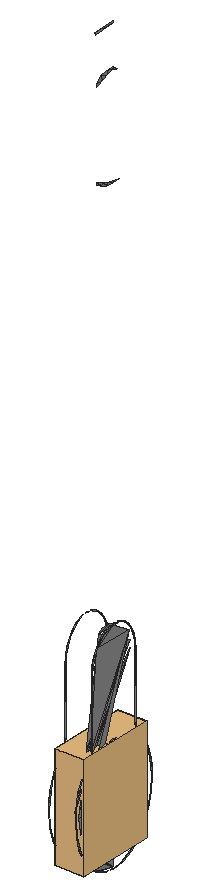
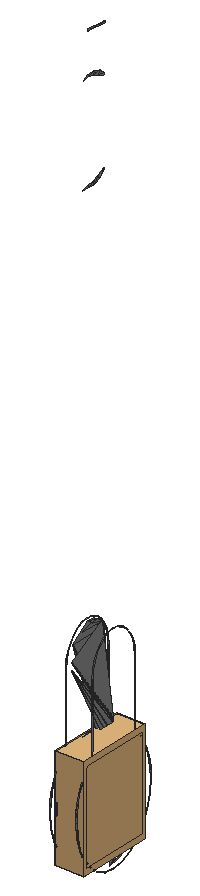
# SketchUp Ruby script. Lengths in inches.
U = 1.inch
M = Sketchup.active_model
def pt(a) = Geom::Point3d.new(a.map { |v| v * U })
def face(e, loops, mat)
  f = e.add_face(loops[0].map { |a| pt(a) })
  loops[1..].each { |l| e.add_face(l.map { |a| pt(a) }).erase! }
  f.material = f.back_material = mat if mat
  f
end
# faces: each face lists its corners as indices into pts; further lists are holes
def faces(e, pts, list, mat = nil) = list.each { |f| face(e, (f[0].is_a?(Array) ? f : [f]).map { |l| l.map { |i| pts[i] } }, mat) }
# xy, xz, yz: faces in a plane at the given z, y or x. An outline is a flat list of corners, or four numbers for a rectangle; further outlines are holes
def ring(l) = l.size == 4 ? [[l[0], l[1]], [l[2], l[1]], [l[2], l[3]], [l[0], l[3]]] : l.each_slice(2).to_a
def flat(e, list, mat, &to3) = list.each { |f| face(e, (f[0].is_a?(Array) ? f : [f]).map { |l| ring(l).map { |u, v| to3.(u, v) } }, mat) }
def xy(e, z, list, mat = nil) = flat(e, list, mat) { |x, y| [x, y, z] }
def xz(e, y, list, mat = nil) = flat(e, list, mat) { |x, z| [x, y, z] }
def yz(e, x, list, mat = nil) = flat(e, list, mat) { |y, z| [x, y, z] }
def lines(e, pts, list) = list.each { |a, b| e.add_line(pt(pts[a]), pt(pts[b])) }
# prism: a flat outline (further loops are holes) pulled along v
def prism(e, loops, v, mat = nil)
  f = face(e, loops, mat); d = Geom::Vector3d.new(v.map { |x| x * U })
  f.pushpull(f.normal.samedirection?(d) ? d.length : -d.length)
end
def box(e, o, s, mat = nil) = prism(e, [[o, [o[0] + s[0], o[1], o[2]], [o[0] + s[0], o[1] + s[1], o[2]], [o[0], o[1] + s[1], o[2]]]], [0, 0, s[2]], mat)
def at(x, y, z, deg = 0) = Geom::Transformation.translation(pt([x, y, z])) * Geom::Transformation.rotation(ORIGIN, Z_AXIS, deg.degrees)
def axes(o, x, y, z) = Geom::Transformation.new([*x, 0, *y, 0, *z, 0, *pt(o).to_a, 1])
def part(name) = M.definitions.add(name)
# library, detail: a bought-in or finely detailed component or shape, given as its bounding box
def library(name, o, s) = part(name).tap { |d| box(d.entities, o, s) }
def detail(e, o, s) = box(e.add_group.entities, o, s)
def put(e, d, t, mat = nil) = e.add_instance(d, t).tap { |i| i.material = mat if mat }
def group(e, t, mat = nil) = e.add_group.tap { |g| g.transformation = t; g.material = mat if mat }.entities
root = M.entities
M.materials.add("Material \#1").color = [140, 140, 140]
c1 = library("3DGeom~13_Defintion",[-84.91,-744.98,-830.03],[169.82,169.83,1000])
c2 = library("3DGeom~12_Defintion",[-95.68,-755.75,-830.03],[191.36,191.37,1000])
c3 = part("3DGeom~10_Defintion")
yz(c3.entities,-68.96,[[-797.08,-844.83,-797.08,-827.59,-922.41,-827.59],[-922.41,-844.83,-797.08,-844.83,-922.41,-827.59]],"Material \#1")
yz(c3.entities,68.97,[[-922.41,-844.83,-797.08,-827.59,-797.08,-844.83],[-922.41,-844.83,-922.41,-827.59,-797.08,-827.59],[-797.08,137.93,-922.41,155.17,-797.08,155.17],[-922.41,137.93,-922.41,155.17,-797.08,137.93]],"Material \#1")
p = [[-15.8,-989.55,-844.83],[-15.8,-989.55,-827.59],[0,-991.38,-827.59],[0,-991.38,-844.83],[15.8,-989.55,-827.59],[15.8,-989.55,-844.83],
  [-30.32,-984.36,-844.83],[-30.32,-984.36,-827.59],[30.31,-984.36,-827.59],[30.31,-984.36,-844.83],[-43.12,-976.21,-844.83],[-43.12,-976.21,-827.59],
  [43.12,-976.21,-827.59],[43.12,-976.21,-844.83],[-53.81,-965.53,-844.83],[-53.81,-965.53,-827.59],[53.8,-965.53,-827.59],[53.8,-965.53,-844.83],
  [-61.95,-952.73,-844.83],[-61.95,-952.73,-827.59],[53.8,-965.53,-827.59],[61.95,-952.73,-827.59],[61.95,-952.73,-844.83],[-67.15,-938.21,-844.83],
  [-67.15,-938.21,-827.59],[67.14,-938.21,-827.59],[67.14,-938.21,-844.83],[-68.96,-922.41,-844.83],[-68.96,-922.41,-827.59],[67.14,-938.21,-827.59],
  [68.97,-922.41,-827.59],[68.97,-922.41,-844.83],[-69.1,-794.86,-844.83],[-69.1,-794.86,-827.59],[-68.96,-797.08,-827.59],[-68.96,-797.08,-844.83],
  [68.97,-797.08,-844.83],[68.97,-797.08,-827.59],[69.11,-794.71,-827.59],[69.11,-794.71,-844.83],[-69.48,-792.73,-844.83],[-69.48,-792.73,-827.59],
  [69.53,-792.51,-827.59],[69.53,-792.51,-844.83],[-70.14,-790.6875,-844.83],[-70.14,-790.6875,-827.59],[70.24,-790.48,-827.59],[70.24,-790.48,-844.83],
  [-71.08,-788.73,-844.83],[-71.08,-788.73,-827.59],[71.22,-788.57,-827.59],[71.22,-788.57,-844.83],[-72.32,-786.86,-844.83],[-72.32,-786.86,-827.59],
  [72.47,-786.78,-827.59],[72.47,-786.78,-844.83],[-73.8,-785.17,-844.83],[-73.8,-785.17,-827.59],[74,-785.04,-827.59],[74,-785.04,-844.83],
  [-75.96,-783.21,-844.83],[-75.96,-783.21,-827.59],[74,-785.04,-827.59],[75.76,-783.39,-827.59],[75.76,-783.39,-844.83],[86.625,-772.95,-827.59],
  [86.61,-772.96,-844.83],[-86.89,-773.25,-844.83],[-86.89,-773.25,-827.59],[-75.96,-783.21,-844.83],[-96.66,-761.8,-844.83],[-96.66,-761.8,-827.59],
  [86.625,-772.95,-827.59],[86.63,-772.94,-844.83],[86.61,-772.96,-844.83],[86.625,-772.95,-827.59],[86.62,-772.95,-827.59],[86.62,-772.95,-827.59],
  [96.31,-761.375,-827.59],[96.31,-761.375,-844.83],[86.63,-772.94,-844.83],[86.625,-772.95,-827.59],[86.62,-772.95,-827.59],[-104.96,-749.18,-844.83],
  [-104.96,-749.18,-827.59],[-96.66,-761.8,-827.59],[-96.66,-761.8,-844.83],[96.31,-761.375,-827.59],[104.62,-748.77,-827.59],[104.62,-748.77,-844.83],
  [-111.64,-735.52,-844.83],[-111.64,-735.52,-827.59],[111.39,-735.21,-827.59],[111.39,-735.21,-844.83],[-116.49,-721.23,-844.83],[-116.49,-721.23,-827.59],
  [116.4375,-720.78,-827.59],[116.4375,-720.78,-844.83],[-119.64,-705.62,-844.83],[-119.64,-705.62,-827.59],[119.6,-705.57,-827.59],[119.6,-705.57,-844.83],
  [-120.6875,-689.65,-844.83],[-120.6875,-689.65,-827.59],[120.69,-689.65,-827.59],[120.69,-689.65,-844.83],[-117.5,-662,-844.83],[-117.5,-662,-827.59],
  [117.5,-662,-827.59],[117.5,-662,-844.83],[-108.41,-636.61,-844.83],[-108.41,-636.61,-827.59],[117.5,-662,-844.83],[108.41,-636.61,-827.59],
  [108.41,-636.61,-844.83],[-93.91,-613.95,-844.83],[-93.91,-613.95,-827.59],[-108.41,-636.61,-827.59],[108.41,-636.61,-844.83],[94.16,-614.19,-827.59],
  [94.16,-614.19,-844.83],[94.16,-614.19,-827.59],[75.46,-595.5,-827.59],[75.46,-595.5,-844.83],[-75.46,-595.5,-844.83],[-75.46,-595.5,-827.59],
  [-93.91,-613.95,-827.59],[-93.91,-613.95,-827.59],[-93.91,-613.95,-844.83],[-53.05,-581.24,-844.83],[-53.05,-581.24,-827.59],[-75.46,-595.5,-827.59],
  [-75.46,-595.5,-844.83],[53.05,-581.24,-827.59],[53.05,-581.24,-844.83],[-27.65,-572.16,-844.83],[-27.65,-572.16,-827.59],[-53.05,-581.24,-827.59],
  [-53.05,-581.24,-844.83],[27.66,-572.16,-827.59],[27.66,-572.16,-844.83],[0,-568.97,-844.83],[0,-568.97,-827.59],[-27.65,-572.16,-827.59],
  [-27.65,-572.16,-844.83],[0,-568.97,-844.83],[-15.8,-989.55,155.17],[0,-991.38,155.17],[0,-991.38,137.93],[-15.8,-989.55,137.93],
  [15.8,-989.55,155.17],[15.8,-989.55,137.93],[-30.32,-984.36,155.17],[-30.32,-984.36,137.93],[30.31,-984.36,155.17],[30.31,-984.36,137.93],
  [-43.125,-976.22,155.17],[-43.125,-976.22,137.93],[43.12,-976.22,155.17],[43.12,-976.22,137.93],[-53.81,-965.53,155.17],[-53.81,-965.53,137.93],
  [53.8,-965.53,155.17],[53.8,-965.53,137.93],[-61.96,-952.73,155.17],[-61.95,-952.73,137.93],[61.95,-952.73,155.17],[61.95,-952.73,137.93],
  [53.8,-965.53,137.93],[-67.15,-938.21,155.17],[-67.15,-938.21,137.93],[67.14,-938.21,155.17],[67.14,-938.21,137.93],[-68.96,-922.41,155.17],
  [-68.96,-922.41,137.93],[68.97,-922.41,155.17],[68.97,-922.41,137.93],[67.14,-938.21,137.93],[-68.97,-797.08,155.17],[-68.97,-797.08,137.93],
  [-69.1,-794.86,155.17],[-69.1,-794.86,137.93],[68.97,-797.08,155.17],[69.11,-794.71,155.17],[69.11,-794.71,137.93],[68.97,-797.08,137.93],
  [-69.48,-792.73,155.17],[-69.48,-792.73,137.93],[69.53,-792.51,155.17],[69.53,-792.51,137.93],[-70.14,-790.6875,155.17],[-70.14,-790.6875,137.93],
  [70.24,-790.48,155.17],[70.24,-790.48,137.93],[-71.08,-788.73,155.17],[-71.08,-788.73,137.93],[71.22,-788.57,155.17],[71.22,-788.57,137.93],
  [-72.32,-786.86,155.17],[-72.32,-786.86,137.93],[72.47,-786.78,155.17],[72.47,-786.78,137.93],[-73.8,-785.17,155.17],[-73.8,-785.17,137.93],
  [74,-785.04,155.17],[74,-785.04,137.93],[-75.96,-783.21,155.17],[-75.96,-783.21,137.93],[75.76,-783.39,155.17],[75.76,-783.39,137.93],
  [74,-785.04,137.93],[86.61,-772.96,155.17],[86.625,-772.95,137.93],[-86.88,-773.25,155.17],[-75.96,-783.21,155.17],[-86.88,-773.25,137.93],
  [-96.66,-761.8,155.17],[-96.66,-761.8,137.93],[86.63,-772.94,155.17],[86.625,-772.95,137.93],[86.61,-772.96,155.17],[86.62,-772.95,137.93],
  [86.625,-772.95,137.93],[96.31,-761.375,155.17],[96.31,-761.375,137.93],[86.62,-772.95,137.93],[86.63,-772.94,155.17],[86.62,-772.95,137.93],
  [86.625,-772.95,137.93],[-104.96,-749.18,155.17],[-96.66,-761.8,155.17],[-96.66,-761.8,137.93],[-104.96,-749.18,137.93],[104.62,-748.77,155.17],
  [104.62,-748.77,137.93],[96.31,-761.375,137.93],[-111.64,-735.52,155.17],[-111.64,-735.52,137.93],[111.39,-735.21,155.17],[111.39,-735.21,137.93],
  [-116.49,-721.23,155.17],[-116.49,-721.23,137.93],[116.4375,-720.78,155.17],[116.4375,-720.78,137.93],[-119.64,-705.62,155.17],[-119.64,-705.62,137.93],
  [119.6,-705.57,155.17],[119.6,-705.57,137.93],[-120.6875,-689.65,155.17],[-120.6875,-689.65,137.93],[120.69,-689.65,155.17],[120.69,-689.65,137.93],
  [-117.5,-662,155.17],[-117.5,-662,137.93],[117.5,-662,155.17],[117.5,-662,137.93],[-108.41,-636.61,155.17],[-108.41,-636.61,137.93],
  [117.5,-662,155.17],[108.41,-636.61,155.17],[108.41,-636.61,137.93],[-93.91,-613.95,155.17],[-108.41,-636.61,137.93],[-93.91,-613.95,137.93],
  [108.41,-636.61,155.17],[94.16,-614.19,155.17],[94.16,-614.19,137.93],[75.46,-595.5,155.17],[75.46,-595.5,137.93],[94.16,-614.19,137.93],
  [-75.46,-595.5,155.17],[-93.91,-613.95,155.17],[-93.91,-613.95,137.93],[-75.46,-595.5,137.93],[-53.05,-581.24,155.17],[-75.46,-595.5,155.17],
  [-75.46,-595.5,137.93],[-53.05,-581.24,137.93],[53.05,-581.24,155.17],[53.05,-581.24,137.93],[-27.65,-572.16,155.17],[-53.05,-581.24,155.17],
  [-53.05,-581.24,137.93],[-27.65,-572.16,137.93],[27.65,-572.16,155.17],[27.65,-572.16,137.93],[0,-568.97,155.17],[-27.65,-572.16,155.17],
  [-27.65,-572.16,137.93],[0,-568.97,137.93],[0,-568.97,155.17]]
faces(c3.entities,p,[[0,1,2],[2,3,0],[3,2,4],[4,5,3],[6,7,1],[1,0,6],[5,4,8],[8,9,5],
  [10,11,7],[7,6,10],[9,8,12],[12,13,9],[14,15,11],[11,10,14],[13,12,16],[16,17,13],
  [18,19,15],[15,14,18],[17,20,21],[21,22,17],[23,24,19],[19,18,23],[22,21,25],[25,26,22],
  [27,28,24],[24,23,27],[26,29,30],[30,31,26],[32,33,34],[34,35,32],[36,37,38],[38,39,36],
  [40,41,33],[33,32,40],[39,38,42],[42,43,39],[44,45,41],[41,40,44],[43,42,46],[46,47,43],
  [48,49,45],[45,44,48],[47,46,50],[50,51,47],[52,53,49],[49,48,52],[51,50,54],[54,55,51],
  [56,57,53],[53,52,56],[55,54,58],[58,59,55],[60,61,57],[57,56,60],[59,62,63],[63,64,59],
  [64,63,65],[65,66,64],[67,68,61],[61,69,67],[70,71,68],[68,67,70],[72,73,66],[74,75,76],
  [73,77,78],[78,79,73],[80,81,82],[83,84,85],[85,86,83],[79,87,88],[88,89,79],[90,91,84],
  [84,83,90],[89,88,92],[92,93,89],[94,95,91],[91,90,94],[93,92,96],[96,97,93],[98,99,95],
  [95,94,98],[97,96,100],[100,101,97],[102,103,99],[99,98,102],[101,100,104],[104,105,101],[106,107,103],
  [103,102,106],[105,104,108],[108,109,105],[110,111,107],[107,106,110],[112,108,113],[113,114,112],[115,116,117],
  [117,110,115],[118,113,119],[119,120,118],[120,121,122],[122,123,120],[124,125,126],[127,128,124],[129,130,131],
  [131,132,129],[123,122,133],[133,134,123],[135,136,137],[137,138,135],[134,133,139],[139,140,134],[141,142,143],
  [143,144,141],[140,139,142],[142,145,140],[146,147,148],[148,149,146],[147,150,151],[151,148,147],[152,146,149],
  [149,153,152],[150,154,155],[155,151,150],[156,152,153],[153,157,156],[154,158,159],[159,155,154],[160,156,157],
  [157,161,160],[158,162,163],[163,159,158],[164,160,161],[161,165,164],[162,166,167],[167,168,162],[169,164,165],
  [165,170,169],[166,171,172],[172,167,166],[173,169,170],[170,174,173],[171,175,176],[176,177,171],[178,173,174],
  [174,179,178],[180,178,179],[179,181,180],[182,183,184],[184,185,182],[186,180,181],[181,187,186],[183,188,189],
  [189,184,183],[190,186,187],[187,191,190],[188,192,193],[193,189,188],[194,190,191],[191,195,194],[192,196,197],
  [197,193,192],[198,194,195],[195,199,198],[196,200,201],[201,197,196],[202,198,199],[199,203,202],[200,204,205],
  [205,201,200],[206,202,203],[203,207,206],[204,208,209],[209,210,204],[208,211,212],[212,209,208],[213,214,207],
  [207,215,213],[216,213,215],[215,217,216],[211,218,219],[220,221,222],[218,223,224],[224,225,218],[226,227,228],
  [229,230,231],[231,232,229],[223,233,234],[234,235,223],[236,229,232],[232,237,236],[233,238,239],[239,234,233],
  [240,236,237],[237,241,240],[238,242,243],[243,239,238],[244,240,241],[241,245,244],[242,246,247],[247,243,242],
  [248,244,245],[245,249,248],[246,250,251],[251,247,246],[252,248,249],[249,253,252],[250,254,255],[255,251,250],
  [256,252,253],[253,257,256],[258,259,260],[260,255,258],[261,256,262],[262,263,261],[264,265,266],[266,260,264],
  [265,267,268],[268,269,265],[270,271,272],[272,273,270],[274,275,276],[276,277,274],[267,278,279],[279,268,267],
  [280,281,282],[282,283,280],[278,284,285],[285,279,278],[286,287,288],[288,289,286],[284,290,289],[289,285,284]],"Material \#1")
xy(root,58.189,[[264.08,328.15,264.104,328.15,264.104,328.205],[264.08,328.15,264.104,328.205,264.08,328.205]],"Material \#1")
xy(root,58.585,[[264.08,328.167,264.08,328.199,264.104,328.167],[264.104,328.167,264.08,328.199,264.104,328.199]],"Material \#1")
xz(root,328.15,[[264.08,58.189,264.08,58.253,264.104,58.189]],"Material \#1")
xz(root,328.156,[[264.08,58.476,264.08,58.513,264.104,58.476]],"Material \#1")
yz(root,263.975,[[328.177,58.05,328.078,58.12,327.978,58.176],[328.177,58.05,328.065,58.084,328.119,58.059],[328.177,58.05,328.177,58.089,328.126,58.097]],"Material \#1")
yz(root,264.078,[[328.177,58.05,327.978,58.176,328.078,58.12],[328.177,58.05,328.119,58.059,328.065,58.084],[328.177,58.05,328.078,58.12,328.126,58.097],[328.177,58.05,328.126,58.097,328.177,58.089],[328.002,58.572,328.029,58.667,328.32,59.055],
  [328.002,58.572,328.32,59.055,328.037,58.619],[328.037,58.619,328.32,59.055,328.078,58.654],[328.078,58.654,328.32,59.055,328.126,58.676],[328.029,58.667,328.032,58.673,328.316,59.098],[328.032,58.673,328.033,58.68,328.316,59.098],
  [328.033,58.68,328.034,58.6875,328.316,59.098],[328.034,58.6875,328.035,58.695,328.316,59.098],[328.035,58.695,328.115,59.224,328.316,59.098],[328.115,59.224,328.145,59.239,328.177,59.244],[328.115,59.224,328.177,59.244,328.24,59.224]],"Material \#1")
yz(root,264.08,[[328.15,58.189,328.205,58.189,328.15,58.253],[328.205,58.189,328.205,58.253,328.15,58.253],[328.15,58.253,328.205,58.253,328.157,58.258],[328.205,58.253,328.198,58.258,328.157,58.258],[328.157,58.258,328.198,58.258,328.157,58.268],
  [328.198,58.258,328.198,58.268,328.157,58.268],[328.157,58.268,328.198,58.268,328.15,58.273],[328.198,58.268,328.205,58.273,328.15,58.273],[328.15,58.273,328.205,58.273,328.15,58.337],[328.205,58.273,328.205,58.337,328.15,58.337],
  [328.15,58.337,328.205,58.337,328.156,58.357],[328.205,58.337,328.199,58.357,328.156,58.357],[328.156,58.357,328.199,58.357,328.148,58.385],[328.199,58.357,328.207,58.385,328.148,58.385],[328.148,58.385,328.207,58.385,328.148,58.413],
  [328.207,58.385,328.207,58.413,328.148,58.413],[328.148,58.413,328.207,58.413,328.156,58.441],[328.207,58.413,328.199,58.441,328.156,58.441],[328.156,58.441,328.199,58.441,328.156,58.476],[328.199,58.441,328.199,58.476,328.156,58.476],
  [328.156,58.476,328.199,58.476,328.156,58.513],[328.199,58.476,328.188,58.513,328.156,58.513],[328.156,58.513,328.188,58.513,328.15,58.523],[328.188,58.513,328.194,58.523,328.15,58.523],[328.15,58.523,328.194,58.523,328.15,58.545],
  [328.194,58.523,328.194,58.545,328.15,58.545],[328.15,58.545,328.194,58.545,328.156,58.555],[328.194,58.545,328.188,58.555,328.156,58.555],[328.156,58.555,328.188,58.555,328.167,58.585],[328.188,58.555,328.199,58.585,328.167,58.585]],"Material \#1")
yz(root,264.098,[[328.177,58.089,328.121,58.109,328.119,58.1],[328.177,58.089,328.177,58.099,328.121,58.109],[328.177,58.089,328.235,58.1,328.177,58.099],[328.177,58.099,328.235,58.1,328.233,58.109],[328.119,58.1,328.069,58.138,328.065,58.129],
  [328.119,58.1,328.121,58.109,328.069,58.138],[328.235,58.1,328.29,58.129,328.233,58.109],[328.233,58.109,328.29,58.129,328.286,58.138],[328.065,58.129,328.023,58.184,328.018,58.177],[328.065,58.129,328.069,58.138,328.023,58.184],
  [328.29,58.129,328.336,58.177,328.286,58.138],[328.286,58.138,328.336,58.177,328.331,58.184],[328.018,58.177,327.989,58.243,327.982,58.238],[328.018,58.177,328.023,58.184,327.989,58.243],[328.336,58.177,328.372,58.238,328.331,58.184],
  [328.331,58.184,328.372,58.238,328.365,58.243],[327.982,58.238,327.967,58.3125,327.96,58.31],[327.982,58.238,327.989,58.243,327.967,58.3125],[328.372,58.238,328.394,58.31,328.365,58.243],[328.365,58.243,328.394,58.31,328.387,58.3125],
  [327.96,58.31,327.96,58.387,327.952,58.387],[327.96,58.31,327.967,58.3125,327.96,58.387],[328.394,58.31,328.402,58.387,328.387,58.3125],[328.387,58.3125,328.402,58.387,328.395,58.387],[327.952,58.387,327.96,58.387,327.967,58.461],
  [327.952,58.387,327.967,58.461,327.96,58.464],[328.395,58.387,328.394,58.464,328.387,58.461],[328.395,58.387,328.402,58.387,328.394,58.464],[327.967,58.461,327.989,58.53,327.96,58.464],[328.387,58.461,328.372,58.535,328.365,58.53],
  [328.387,58.461,328.394,58.464,328.372,58.535],[327.96,58.464,327.989,58.53,327.982,58.535],[327.989,58.53,328.023,58.59,327.982,58.535],[328.365,58.53,328.336,58.597,328.331,58.59],[328.365,58.53,328.372,58.535,328.336,58.597],
  [327.982,58.535,328.023,58.59,328.018,58.597],[328.023,58.59,328.069,58.635,328.018,58.597],[328.331,58.59,328.29,58.644,328.286,58.635],[328.331,58.59,328.336,58.597,328.29,58.644],[328.018,58.597,328.069,58.635,328.065,58.644],
  [328.069,58.635,328.121,58.664,328.065,58.644],[328.286,58.635,328.235,58.674,328.233,58.664],[328.286,58.635,328.29,58.644,328.235,58.674],[328.065,58.644,328.121,58.664,328.119,58.674],[328.121,58.664,328.177,58.674,328.119,58.674],
  [328.233,58.664,328.177,58.684,328.177,58.674],[328.233,58.664,328.235,58.674,328.177,58.684],[328.119,58.674,328.177,58.674,328.177,58.684]],"Material \#1")
yz(root,264.101,[[328.177,61.418,328.14,61.437,328.138,61.422],[328.177,61.418,328.177,61.432,328.14,61.437],[328.177,61.418,328.216,61.422,328.177,61.432],[328.138,61.422,328.105,61.45,328.101,61.436],[328.138,61.422,328.14,61.437,328.105,61.45],
  [328.101,61.436,328.073,61.47,328.067,61.457],[328.101,61.436,328.105,61.45,328.073,61.47],[328.073,61.941,328.105,61.961,328.067,61.954],[328.067,61.954,328.105,61.961,328.101,61.975],[328.105,61.961,328.14,61.974,328.101,61.975],
  [328.14,61.974,328.138,61.989,328.101,61.975],[328.14,61.974,328.177,61.978,328.138,61.989],[328.214,61.974,328.177,61.993,328.177,61.978],[328.177,61.978,328.177,61.993,328.138,61.989],[328.061,62.196,328.177,62.21,328.059,62.211],
  [328.177,62.21,328.177,62.225,328.059,62.211]],"Material \#1")
yz(root,264.103,[[328.177,58.05,327.978,58.176,328.065,58.084],[328.177,58.05,328.078,58.12,327.978,58.176],[328.177,58.05,328.065,58.084,328.119,58.059],[328.177,58.05,328.126,58.097,328.078,58.12],[328.177,58.05,328.177,58.089,328.126,58.097],
  [327.924,58.431,328.288,59.173,328.029,58.667],[328.078,58.654,328.126,58.676,328.288,59.173],[328.034,58.6875,328.288,59.173,328.066,59.173],[328.066,59.173,328.115,59.224,328.088,59.202],[328.066,59.173,328.177,59.244,328.115,59.224],
  [328.066,59.173,328.288,59.173,328.177,59.244],[328.115,59.224,328.177,59.244,328.145,59.239]],"Material \#1")
yz(root,264.104,[[328.177,58.122,328.127,58.14,328.125,58.131],[328.177,58.122,328.177,58.132,328.127,58.14],[328.177,58.122,328.229,58.131,328.177,58.132],[328.125,58.131,328.081,58.166,328.077,58.157],[328.125,58.131,328.127,58.14,328.081,58.166],
  [328.229,58.131,328.227,58.14,328.177,58.132],[328.229,58.131,328.277,58.157,328.227,58.14],[328.227,58.14,328.277,58.157,328.274,58.166],[328.077,58.157,328.041,58.206,328.035,58.199],[328.077,58.157,328.081,58.166,328.041,58.206],
  [328.277,58.157,328.319,58.199,328.274,58.166],[328.274,58.166,328.319,58.199,328.314,58.206],[328.035,58.199,328.01,58.259,328.004,58.254],[328.035,58.199,328.041,58.206,328.01,58.259],[328.319,58.199,328.351,58.254,328.314,58.206],
  [328.314,58.206,328.351,58.254,328.344,58.259],[328.004,58.254,327.991,58.321,327.984,58.318],[328.004,58.254,328.01,58.259,327.991,58.321],[328.351,58.254,328.371,58.318,328.344,58.259],[328.344,58.259,328.371,58.318,328.364,58.321],
  [327.984,58.318,327.984,58.387,327.977,58.387],[327.984,58.318,327.991,58.321,327.984,58.387],[328.371,58.318,328.378,58.387,328.364,58.321],[328.364,58.321,328.378,58.387,328.37,58.387],[327.977,58.387,327.984,58.387,327.991,58.453],
  [327.977,58.387,327.991,58.453,327.984,58.455],[328.37,58.387,328.371,58.455,328.364,58.453],[328.37,58.387,328.378,58.387,328.371,58.455],[327.991,58.453,328.01,58.514,327.984,58.455],[328.364,58.453,328.351,58.519,328.344,58.514],
  [328.364,58.453,328.371,58.455,328.351,58.519],[327.984,58.455,328.01,58.514,328.004,58.519],[328.01,58.514,328.041,58.567,328.004,58.519],[328.344,58.514,328.319,58.574,328.314,58.567],[328.344,58.514,328.351,58.519,328.319,58.574],
  [328.004,58.519,328.041,58.567,328.035,58.574],[328.041,58.567,328.081,58.607,328.035,58.574],[328.314,58.567,328.277,58.616,328.274,58.607],[328.314,58.567,328.319,58.574,328.277,58.616],[328.035,58.574,328.081,58.607,328.077,58.616],
  [328.081,58.607,328.127,58.633,328.077,58.616],[328.274,58.607,328.229,58.643,328.227,58.633],[328.274,58.607,328.277,58.616,328.229,58.643],[328.077,58.616,328.127,58.633,328.125,58.643],[328.127,58.633,328.177,58.642,328.125,58.643],
  [328.227,58.633,328.177,58.652,328.177,58.642],[328.227,58.633,328.229,58.643,328.177,58.652],[328.177,58.642,328.177,58.652,328.125,58.643]],"Material \#1")
p = [[264.08,328.15,58.253],[264.104,328.153,58.267],[264.104,328.15,58.189],[264.104,328.153,58.347],[264.08,328.156,58.357],[264.08,328.148,58.385],
  [264.08,328.148,58.385],[264.104,328.152,58.371],[264.104,328.153,58.347],[264.104,328.202,58.261],[264.08,328.205,58.273],[264.08,328.198,58.268],
  [264.104,328.153,58.267],[264.08,328.157,58.258],[264.08,328.157,58.268],[264.104,328.153,58.267],[264.08,328.15,58.253],[264.104,328.153,58.267],
  [264.08,328.15,58.273],[264.104,328.202,58.261],[264.08,328.198,58.258],[264.08,328.205,58.253],[264.104,328.202,58.261],[264.104,328.15,58.333],
  [264.08,328.15,58.337],[264.08,328.156,58.357],[264.104,328.153,58.267],[264.08,328.15,58.273],[264.08,328.15,58.337],[264.08,328.156,58.357],
  [264.104,328.153,58.347],[264.104,328.15,58.333],[264.08,328.15,58.337],[264.104,328.15,58.333],[264.104,328.153,58.267],[264.104,328.152,58.371],
  [264.08,328.148,58.385],[264.08,328.148,58.413],[264.104,328.148,58.399],[264.08,328.148,58.413],[264.08,328.156,58.441],[264.08,328.148,58.413],
  [264.104,328.148,58.399],[264.104,328.152,58.371],[264.08,328.156,58.441],[264.104,328.152,58.427],[264.104,328.148,58.399],[264.104,328.152,58.427],
  [264.08,328.156,58.441],[264.08,328.156,58.476],[264.08,328.156,58.476],[264.104,328.156,58.476],[264.104,328.152,58.427],[264.104,328.191,58.55],
  [264.08,328.188,58.555],[264.08,328.194,58.545],[264.104,328.191,58.518],[264.08,328.194,58.523],[264.08,328.188,58.513],[264.104,328.153,58.55],
  [264.08,328.15,58.545],[264.08,328.156,58.555],[264.104,328.153,58.518],[264.08,328.156,58.513],[264.08,328.15,58.523],[264.104,328.153,58.518],
  [264.08,328.15,58.523],[264.08,328.15,58.545],[264.104,328.153,58.55],[264.08,328.156,58.513],[264.104,328.153,58.518],[264.104,328.156,58.476],
  [264.104,328.153,58.55],[264.08,328.156,58.555],[264.08,328.167,58.585],[264.104,328.167,58.585],[264.104,328.153,58.55],[264.101,328.196,61.611],
  [264.099,328.196,61.611],[264.099,328.117,61.761],[264.101,328.117,61.761],[264.101,328.238,61.65],[264.099,328.238,61.65],[264.099,328.252,61.622],
  [264.101,328.252,61.622],[264.1,328.269,61.591],[264.098,328.269,61.591],[264.098,328.25,61.568],[264.1,328.25,61.568],[264.098,328.227,61.552],
  [264.1,328.227,61.552],[264.099,328.211,61.583],[264.101,328.211,61.583],[264.101,328.158,61.8],[264.099,328.158,61.8],[264.099,328.102,61.789],
  [264.101,328.102,61.789],[264.098,328.085,61.82],[264.1,328.085,61.82],[264.098,328.104,61.843],[264.1,328.104,61.843],[264.098,328.127,61.858],
  [264.1,328.127,61.858],[264.099,328.144,61.827],[264.101,328.144,61.827]]
faces(root,p,[[0,1,2],[3,4,5],[6,7,8],[9,10,11],[12,13,14],[15,16,13],[17,14,18],[19,20,21],
  [22,11,20],[23,24,25],[26,27,28],[29,30,31],[32,33,34],[35,36,37],[38,39,40],[41,42,43],
  [44,45,46],[47,48,49],[50,51,52],[53,54,55],[56,57,58],[59,60,61],[62,63,64],[65,66,67],
  [67,68,65],[69,70,71],[72,73,74],[74,75,76],[77,78,79],[79,80,77],[81,82,83],[83,84,81],
  [85,86,87],[87,88,85],[88,87,89],[89,90,88],[90,89,91],[91,92,90],[92,91,78],[78,77,92],
  [93,94,82],[82,81,93],[84,83,86],[86,85,84],[80,79,95],[95,96,80],[96,95,97],[97,98,96],
  [98,97,99],[99,100,98],[100,99,101],[101,102,100],[102,101,103],[103,104,102],[104,103,94],[94,93,104]],"Material \#1")
put(root,c1,axes([263.98,328.18,56.41],[0,0.00227,0],[0,0,-0.003],[-0.00016,0,0]),"Material \#1")
put(root,c2,axes([263.98,328.18,56.41],[0,0.00227,0],[0,0,-0.003],[-0.00016,0,0]),"Material \#1")
put(root,c3,axes([263.98,328.18,56.41],[0,0.00217,0],[0,0,-0.00287],[-0.00015,0,0]),"Material \#1")
